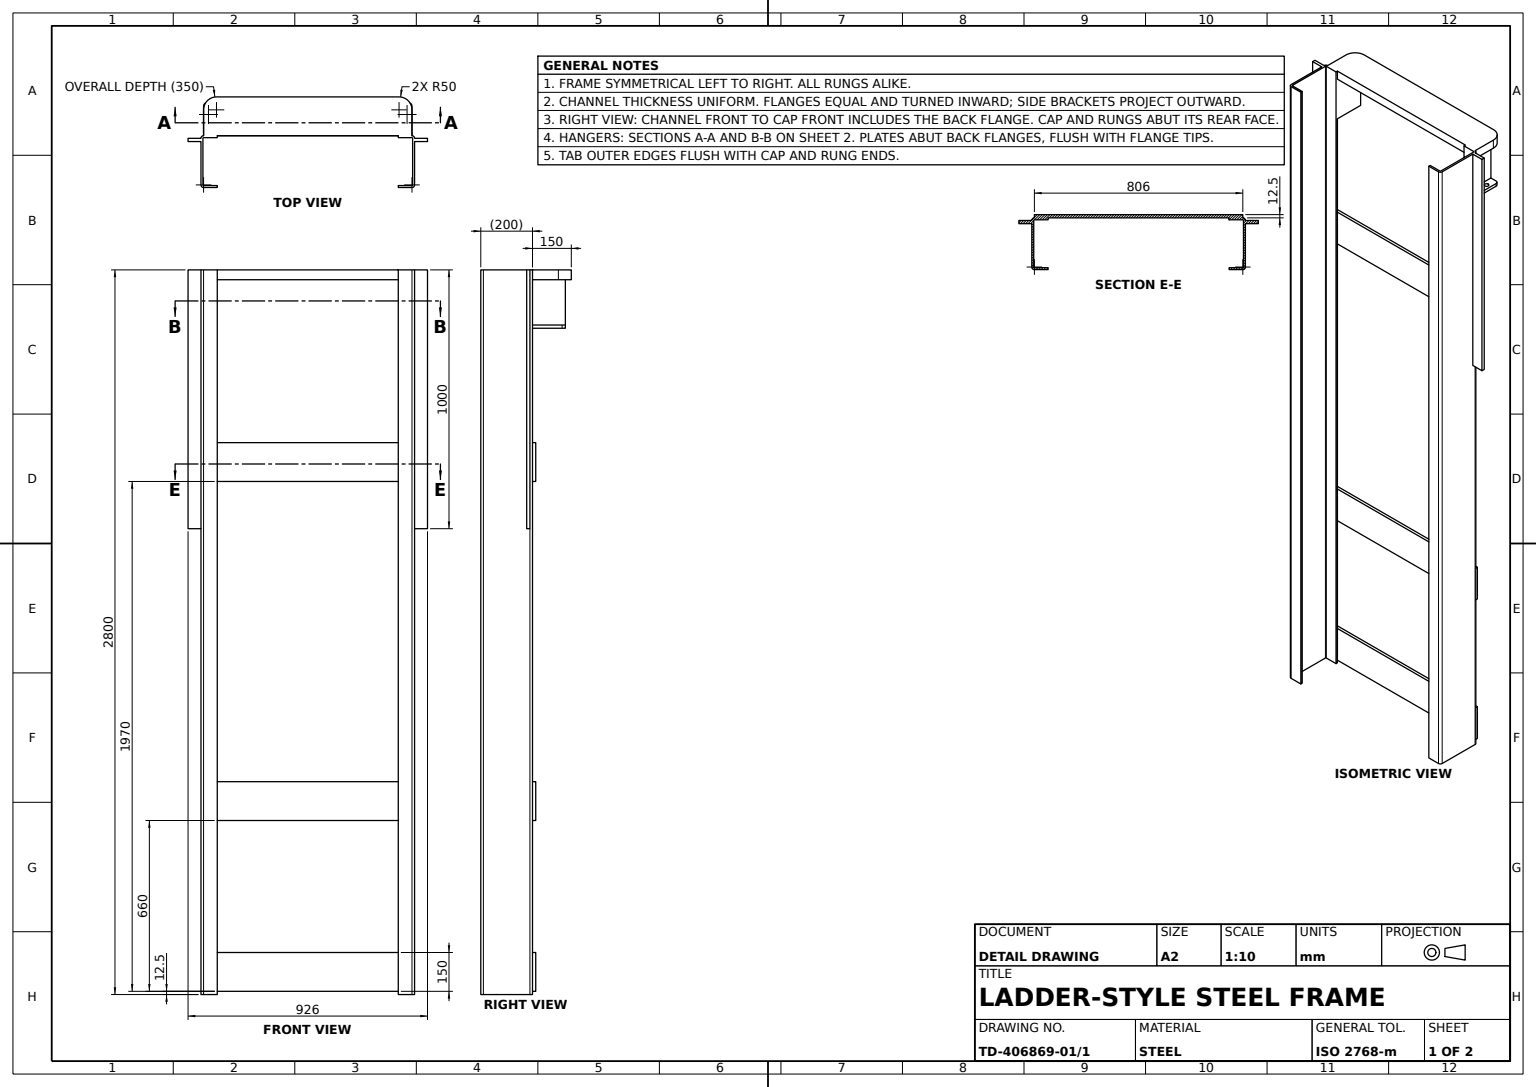
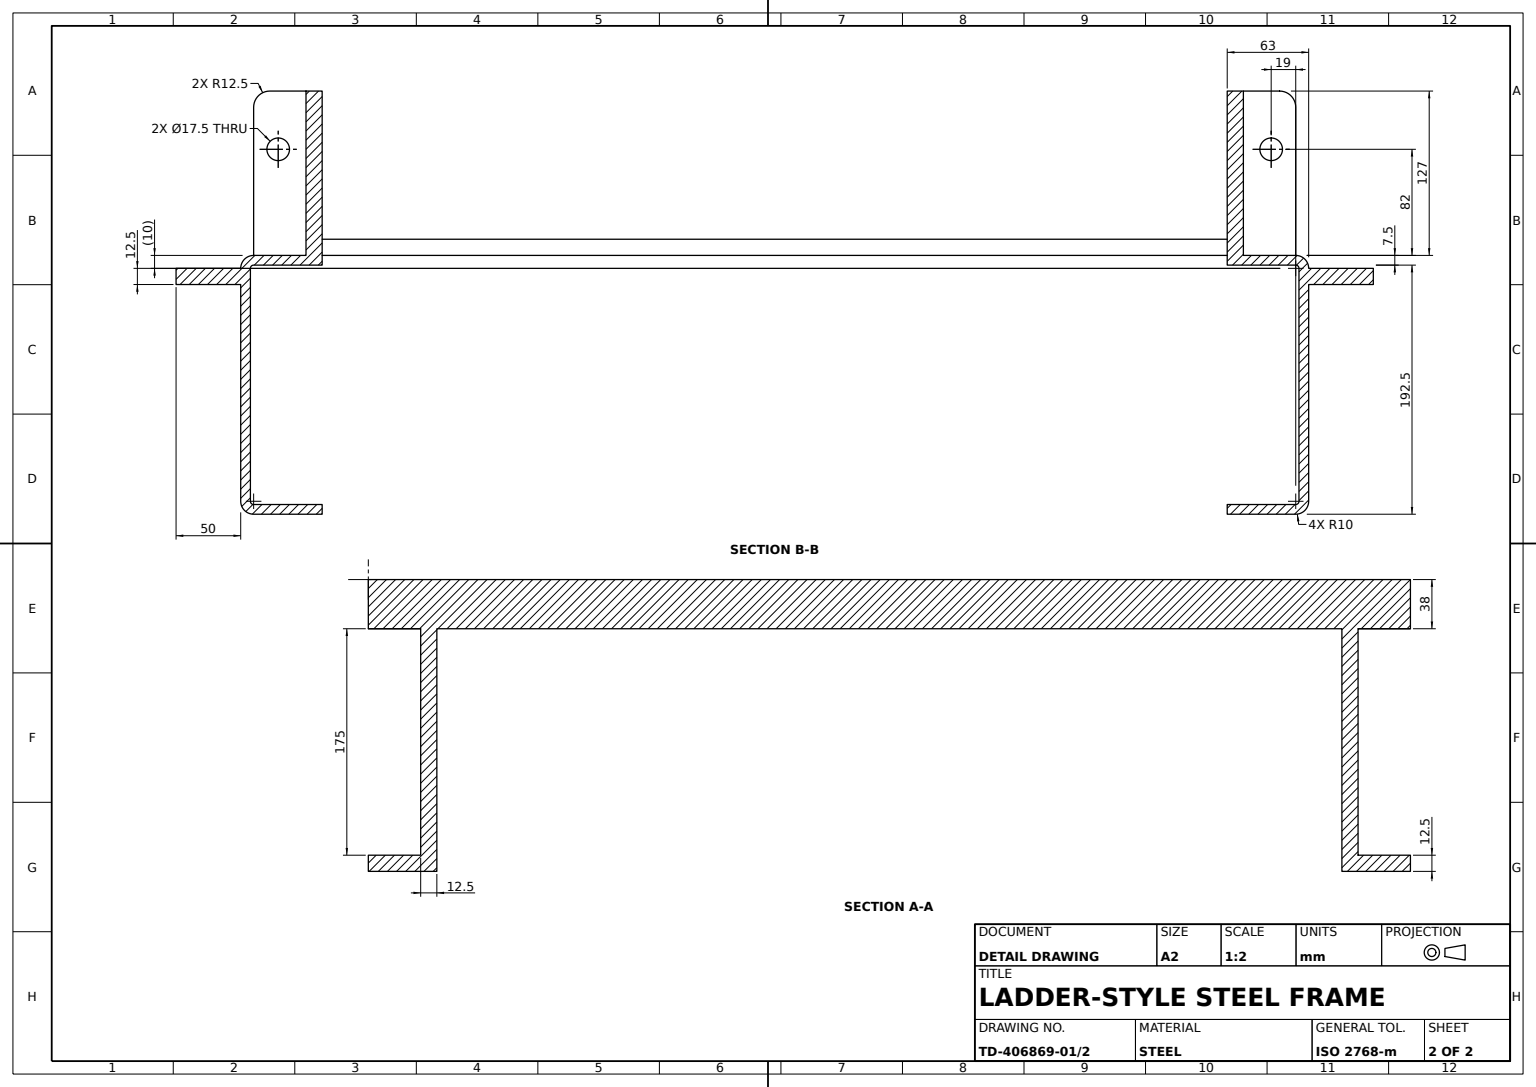
solid
v1 (-403,1400,-200)
v2 (-403,1400,-100)
e1 v1 v2 LINE
v3 (-403,1362,-200)
e2 v3 v1 LINE
v4 (-403,1362,-100)
e3 v3 v4 LINE
e4 v4 v2 LINE
face PLANE(AX(P(-403,1362,-100),D(-1,0,0),D(0,0,1))) [-e1 -e2 e3 e4]
v5 (-350,-1237.5,-100)
v6 (350,-1237.5,-100)
e5 v5 v6 LINE
v7 (-350,-1387.5,-100)
e6 v5 v7 LINE
v8 (350,-1387.5,-100)
e7 v8 v7 LINE
e8 v8 v6 LINE
face PLANE(AX(P(0,0,-100),D(0,0,1),D(1,0,0))) [-e5 e6 -e7 e8]
v9 (384,1174.5,-173.25)
v10 (384,1187,-173.25)
e9 v9 v10 LINE
v11 (384,1187,-190.75)
e10 v10 v11 CIRCLE(AX(P(384,1187,-182),D(0,1,0),D(0,0,-1)),8.75)
v12 (384,1174.5,-190.75)
e11 v12 v11 LINE
e12 v9 v12 CIRCLE(AX(P(384,1174.5,-182),D(0,1,0),D(0,0,-1)),8.75)
face CYL(AX(P(384,1174.5,-182),D(0,1,0),D(0,0,1)),8.75) rev [e9 e10 -e11 -e12]
v13 (350,-727.5,-100)
e13 v13 v6 LINE
v14 (403,-727.5,-100)
e14 v14 v13 LINE
v15 (403,-1237.5,-100)
e15 v14 v15 LINE
e16 v6 v15 LINE
face PLANE(AX(P(350,1400,-100),D(0,0,-1),D(-1,0,0))) [-e13 -e14 e15 -e16]
v16 (-384,1174.5,-173.25)
v17 (-384,1187,-173.25)
e17 v16 v17 LINE
v18 (-384,1174.5,-190.75)
e18 v16 v18 CIRCLE(AX(P(-384,1174.5,-182),D(0,-1,0),D(0,0,-1)),8.75)
v19 (-384,1187,-190.75)
e19 v18 v19 LINE
e20 v17 v19 CIRCLE(AX(P(-384,1187,-182),D(0,-1,0),D(0,0,-1)),8.75)
face CYL(AX(P(-384,1174.5,-182),D(0,1,0),D(0,0,1)),8.75) rev [-e17 e18 e19 -e20]
v20 (390.5,1187,-227)
v21 (362.5,1187,-227)
e21 v20 v21 LINE
v22 (362.5,1187,-100)
e22 v22 v21 LINE
v23 (403,1187,-100)
e23 v22 v23 LINE
v24 (403,1187,-214.5)
e24 v23 v24 LINE
e25 v20 v24 CIRCLE(AX(P(390.5,1187,-214.5),D(0,-1,0),D(0,0,1)),12.5)
e26 v11 v10 CIRCLE(AX(P(384,1187,-182),D(0,1,0),D(0,0,-1)),8.75)
face PLANE(AX(P(0,1187,0),D(0,1,0),D(0,0,1))) [e21 -e22 e23 e24 -e25] [-e26 -e10]
v25 (350,1400,92.5)
v26 (350,-1400,92.5)
e27 v25 v26 LINE
v27 (403,1400,92.5)
e28 v27 v25 LINE
v28 (403,-1400,92.5)
e29 v27 v28 LINE
e30 v28 v26 LINE
face PLANE(AX(P(403,1400,92.5),D(0,0,1),D(1,0,0))) rev [-e27 -e28 e29 e30]
v29 (405.5,1400,90)
e31 v29 v27 CIRCLE(AX(P(403,1400,90),D(0,-1,0),D(1,0,0)),2.5)
v30 (405.5,-1400,90)
e32 v29 v30 LINE
e33 v30 v28 CIRCLE(AX(P(403,-1400,90),D(0,-1,0),D(1,0,0)),2.5)
face CYL(AX(P(403,1400,90),D(0,-1,0),D(0,0,-1)),2.5) rev [-e29 -e31 e32 e33]
v31 (403,1362,-200)
v32 (353,1362,-250)
e34 v31 v32 CIRCLE(AX(P(353,1362,-200),D(0,1,0),D(0,0,-1)),50)
v33 (353,1400,-250)
e35 v32 v33 LINE
v34 (403,1400,-200)
e36 v34 v33 CIRCLE(AX(P(353,1400,-200),D(0,1,0),D(0,0,-1)),50)
e37 v31 v34 LINE
face CYL(AX(P(353,1362,-200),D(0,1,0),D(0,0,1)),50) [e34 e35 -e36 -e37]
v35 (-403,-577.5,-112.5)
v36 (403,-577.5,-112.5)
e38 v35 v36 LINE
v37 (403,-727.5,-112.5)
e39 v36 v37 LINE
v38 (-403,-727.5,-112.5)
e40 v37 v38 LINE
e41 v38 v35 LINE
face PLANE(AX(P(0,660,-112.5),D(0,0,1),D(1,0,0))) rev [e38 e39 e40 e41]
v39 (403,732.5,-112.5)
v40 (403,732.5,-100)
e42 v39 v40 LINE
v41 (403,582.5,-100)
e43 v40 v41 LINE
v42 (403,582.5,-112.5)
e44 v42 v41 LINE
e45 v39 v42 LINE
face PLANE(AX(P(403,582.5,-112.5),D(-1,0,0),D(0,0,1))) rev [e42 e43 -e44 -e45]
v43 (-403,-1237.5,-112.5)
v44 (-403,-1237.5,-100)
e46 v43 v44 LINE
e47 v44 v5 LINE
v45 (403,-1237.5,-112.5)
e48 v45 v15 LINE
e49 v43 v45 LINE
face PLANE(AX(P(403,-1237.5,-112.5),D(0,-1,0),D(0,0,-1))) rev [e46 e47 e5 e16 -e48 -e49]
v46 (-403,-1387.5,-112.5)
v47 (-403,-1387.5,-100)
e50 v46 v47 LINE
e51 v47 v44 LINE
e52 v46 v43 LINE
face PLANE(AX(P(-403,-1387.5,-112.5),D(1,0,0),D(0,0,-1))) rev [e50 e51 -e46 -e52]
v48 (413,-1400,90)
v49 (403,-1400,100)
e53 v48 v49 CIRCLE(AX(P(403,-1400,90),D(0,-1,0),D(0,0,-1)),10)
v50 (413,1400,90)
e54 v50 v48 LINE
v51 (403,1400,100)
e55 v50 v51 CIRCLE(AX(P(403,1400,90),D(0,-1,0),D(0,0,-1)),10)
e56 v51 v49 LINE
face CYL(AX(P(403,1400,90),D(0,-1,0),D(0,0,-1)),10) [-e53 -e54 e55 e56]
v52 (-350,-727.5,-100)
e57 v52 v5 LINE
v53 (-403,-727.5,-100)
e58 v53 v44 LINE
e59 v52 v53 LINE
face PLANE(AX(P(-350,1400,-100),D(0,0,-1),D(1,0,0))) [e57 -e47 -e58 -e59]
e60 v37 v14 LINE
v54 (403,-577.5,-100)
e61 v36 v54 LINE
e62 v54 v14 LINE
face PLANE(AX(P(403,-727.5,-112.5),D(-1,0,0),D(0,0,1))) rev [-e60 -e39 e61 e62]
v55 (-403,1400,92.5)
v56 (-403,-1400,92.5)
e63 v55 v56 LINE
v57 (-405.5,-1400,90)
e64 v57 v56 CIRCLE(AX(P(-403,-1400,90),D(0,1,0),D(-1,0,0)),2.5)
v58 (-405.5,1400,90)
e65 v58 v57 LINE
e66 v58 v55 CIRCLE(AX(P(-403,1400,90),D(0,1,0),D(-1,0,0)),2.5)
face CYL(AX(P(-403,1400,90),D(0,-1,0),D(0,0,-1)),2.5) rev [e63 -e64 -e65 e66]
e67 v38 v53 LINE
v59 (-403,-577.5,-100)
e68 v53 v59 LINE
e69 v35 v59 LINE
face PLANE(AX(P(-403,-727.5,-112.5),D(1,0,0),D(0,0,-1))) rev [-e41 e67 e68 -e69]
e70 v12 v9 CIRCLE(AX(P(384,1174.5,-182),D(0,1,0),D(0,0,-1)),8.75)
face CYL(AX(P(384,1174.5,-182),D(0,1,0),D(0,0,1)),8.75) rev [-e70 e11 e26 -e9]
e71 v18 v16 CIRCLE(AX(P(-384,1174.5,-182),D(0,-1,0),D(0,0,-1)),8.75)
e72 v19 v17 CIRCLE(AX(P(-384,1187,-182),D(0,-1,0),D(0,0,-1)),8.75)
face CYL(AX(P(-384,1174.5,-182),D(0,1,0),D(0,0,1)),8.75) rev [e71 e17 -e72 -e19]
v60 (-390.5,1187,-227)
v61 (-403,1187,-214.5)
e73 v60 v61 CIRCLE(AX(P(-390.5,1187,-214.5),D(0,1,0),D(0,0,1)),12.5)
v62 (-390.5,1174.5,-227)
e74 v62 v60 LINE
v63 (-403,1174.5,-214.5)
e75 v63 v62 CIRCLE(AX(P(-390.5,1174.5,-214.5),D(0,-1,0),D(0,0,1)),12.5)
e76 v61 v63 LINE
face CYL(AX(P(-390.5,1187,-214.5),D(0,1,0),D(0,0,1)),12.5) [-e73 -e74 -e75 -e76]
v64 (413,-1400,-90)
e77 v64 v48 LINE
v65 (413,400,-90)
e78 v65 v64 LINE
v66 (413,400,-77.5)
e79 v65 v66 LINE
v67 (413,1400,-77.5)
e80 v66 v67 LINE
e81 v67 v50 LINE
face PLANE(AX(P(413,1400,-90),D(1,0,0),D(0,0,-1))) [-e77 -e78 e79 e80 e81 e54]
v68 (403,-1400,-92.5)
v69 (405.5,-1400,-90)
e82 v68 v69 CIRCLE(AX(P(403,-1400,-90),D(0,-1,0),D(1,0,0)),2.5)
v70 (405.5,1400,-90)
e83 v70 v69 LINE
v71 (403,1400,-92.5)
e84 v71 v70 CIRCLE(AX(P(403,1400,-90),D(0,-1,0),D(1,0,0)),2.5)
e85 v71 v68 LINE
face CYL(AX(P(403,1400,-90),D(0,-1,0),D(0,0,-1)),2.5) rev [e82 -e83 -e84 e85]
v72 (350,582.5,-100)
v73 (350,732.5,-100)
e86 v72 v73 LINE
v74 (-350,732.5,-100)
e87 v74 v73 LINE
v75 (-350,582.5,-100)
e88 v74 v75 LINE
e89 v72 v75 LINE
face PLANE(AX(P(0,1970,-100),D(0,0,1),D(1,0,0))) [e86 -e87 e88 -e89]
v76 (403,1362,-100)
e90 v76 v31 LINE
v77 (403,1400,-100)
e91 v77 v34 LINE
e92 v77 v76 LINE
face PLANE(AX(P(403,1362,-100),D(1,0,0),D(0,0,-1))) [e90 e37 -e91 e92]
v78 (403,-1387.5,-100)
e93 v78 v8 LINE
v79 (403,-1400,-100)
e94 v78 v79 LINE
v80 (350,-1400,-100)
e95 v80 v79 LINE
e96 v8 v80 LINE
face PLANE(AX(P(350,1400,-100),D(0,0,-1),D(-1,0,0))) [-e93 e94 -e95 -e96]
v81 (403,-1387.5,-112.5)
e97 v81 v46 LINE
e98 v45 v81 LINE
face PLANE(AX(P(0,0,-112.5),D(0,0,1),D(1,0,0))) rev [e97 e52 e49 e98]
v82 (362.5,1362,-100)
e99 v82 v76 LINE
v83 (362.5,1362,-227)
e100 v82 v83 LINE
v84 (350,1362,-227)
e101 v83 v84 LINE
v85 (350,1362,-100)
e102 v84 v85 LINE
v86 (-350,1362,-100)
e103 v86 v85 LINE
v87 (-350,1362,-227)
e104 v87 v86 LINE
v88 (-362.5,1362,-227)
e105 v88 v87 LINE
v89 (-362.5,1362,-100)
e106 v89 v88 LINE
e107 v4 v89 LINE
v90 (-353,1362,-250)
e108 v90 v3 CIRCLE(AX(P(-353,1362,-200),D(0,1,0),D(0,0,-1)),50)
e109 v32 v90 LINE
face PLANE(AX(P(-353,1362,-200),D(0,-1,0),D(0,0,-1))) [-e90 -e99 e100 e101 e102 -e103 -e104 -e105 -e106 -e107 -e3 -e108 -e109 -e34]
v91 (-350,1174.5,-227)
v92 (-350,1174.5,-100)
e110 v91 v92 LINE
v93 (-403,1174.5,-100)
e111 v92 v93 LINE
e112 v93 v63 LINE
e113 v62 v91 LINE
face PLANE(AX(P(0,1174.5,0),D(0,1,0),D(0,0,1))) rev [e110 e111 e112 e75 e113] [-e18 -e71]
v94 (-350,1400,-100)
e114 v94 v86 LINE
v95 (350,1400,-100)
e115 v95 v85 LINE
e116 v94 v95 LINE
face PLANE(AX(P(-403,1362,-100),D(0,0,1),D(1,0,0))) [e114 e103 -e115 -e116]
v96 (-353,1400,-250)
e117 v96 v1 CIRCLE(AX(P(-353,1400,-200),D(0,1,0),D(0,0,-1)),50)
e118 v90 v96 LINE
face CYL(AX(P(-353,1362,-200),D(0,1,0),D(0,0,1)),50) [e108 e2 -e117 -e118]
v97 (-405.5,1400,-90)
e119 v97 v58 LINE
v98 (-405.5,-1400,-90)
e120 v98 v57 LINE
e121 v97 v98 LINE
face PLANE(AX(P(-405.5,1400,-90),D(-1,0,0),D(0,0,-1))) rev [e119 e65 -e120 -e121]
v99 (350,-1400,-92.5)
e122 v99 v80 LINE
e123 v79 v64 CIRCLE(AX(P(403,-1400,-90),D(0,-1,0),D(0,0,-1)),10)
v100 (350,-1400,100)
e124 v49 v100 LINE
e125 v100 v26 LINE
e126 v69 v30 LINE
e127 v99 v68 LINE
face PLANE(AX(P(403,-1400,90),D(0,-1,0),D(-1,0,0))) [e122 e95 e123 e77 e53 e124 e125 -e30 -e33 -e126 -e82 -e127]
v101 (403,1174.5,-214.5)
e128 v24 v101 LINE
v102 (390.5,1174.5,-227)
e129 v101 v102 CIRCLE(AX(P(390.5,1174.5,-214.5),D(0,1,0),D(0,0,1)),12.5)
e130 v102 v20 LINE
face CYL(AX(P(390.5,1187,-214.5),D(0,1,0),D(0,0,1)),12.5) [e25 e128 e129 e130]
v103 (350,-577.5,-100)
e131 v103 v54 LINE
e132 v72 v103 LINE
e133 v41 v72 LINE
e134 v41 v54 LINE
face PLANE(AX(P(350,1400,-100),D(0,0,-1),D(-1,0,0))) [-e131 -e132 -e133 e134]
v104 (463,400,-77.5)
v105 (463,1400,-77.5)
e135 v104 v105 LINE
v106 (463,400,-90)
e136 v104 v106 LINE
v107 (463,1400,-90)
e137 v106 v107 LINE
e138 v105 v107 LINE
face PLANE(AX(P(463,400,-90),D(1,0,0),D(0,0,-1))) [-e135 e136 e137 -e138]
e139 v21 v83 LINE
v108 (350,1174.5,-227)
e140 v102 v108 LINE
e141 v108 v84 LINE
face PLANE(AX(P(350,1187,-227),D(0,0,1),D(-1,0,0))) rev [-e139 -e21 -e130 e140 e141 -e101]
v109 (-403,582.5,-100)
e142 v75 v109 LINE
v110 (-350,-577.5,-100)
e143 v75 v110 LINE
e144 v59 v110 LINE
e145 v109 v59 LINE
face PLANE(AX(P(-350,1400,-100),D(0,0,-1),D(1,0,0))) [-e142 e143 -e144 -e145]
e146 v13 v52 LINE
face PLANE(AX(P(403,-727.5,-112.5),D(0,1,0),D(0,0,1))) rev [e14 e146 e59 -e67 -e40 e60]
v111 (-403,-1400,-100)
e147 v47 v111 LINE
v112 (-413,-1400,-90)
e148 v111 v112 CIRCLE(AX(P(-403,-1400,-90),D(0,1,0),D(0,0,-1)),10)
v113 (-413,400,-90)
e149 v113 v112 LINE
v114 (-413,1400,-90)
e150 v114 v113 LINE
e151 v2 v114 CIRCLE(AX(P(-403,1400,-90),D(0,1,0),D(0,0,-1)),10)
v115 (-403,1187,-100)
e152 v4 v115 LINE
e153 v93 v115 LINE
v116 (-403,732.5,-100)
e154 v93 v116 LINE
e155 v109 v116 LINE
face CYL(AX(P(-403,1400,-90),D(0,-1,0),D(0,0,-1)),10) [e145 -e68 e58 -e51 e147 e148 -e149 -e150 -e151 -e4 e152 -e153 e154 -e155]
v117 (350,1174.5,-100)
e156 v108 v117 LINE
v118 (403,1174.5,-100)
e157 v118 v101 LINE
e158 v117 v118 LINE
face PLANE(AX(P(0,1174.5,0),D(0,1,0),D(0,0,1))) rev [-e156 -e140 -e129 -e157 -e158] [e70 e12]
v119 (-413,1400,-77.5)
v120 (-463,1400,-77.5)
e159 v119 v120 LINE
v121 (-463,400,-77.5)
e160 v121 v120 LINE
v122 (-413,400,-77.5)
e161 v122 v121 LINE
e162 v122 v119 LINE
face PLANE(AX(P(-463,400,-77.5),D(0,0,1),D(-1,0,0))) [e159 -e160 -e161 e162]
e163 v115 v61 LINE
face PLANE(AX(P(-403,1174.5,-100),D(1,0,0),D(0,0,-1))) rev [e163 e76 -e112 e153]
e164 v67 v105 LINE
e165 v66 v104 LINE
face PLANE(AX(P(463,400,-77.5),D(0,0,1),D(1,0,0))) [e135 -e164 -e80 e165]
v123 (-403,-1400,100)
v124 (-350,-1400,100)
e166 v123 v124 LINE
v125 (-350,1400,100)
e167 v125 v124 LINE
v126 (-403,1400,100)
e168 v126 v125 LINE
e169 v126 v123 LINE
face PLANE(AX(P(-403,1400,100),D(0,0,1),D(-1,0,0))) [e166 -e167 -e168 e169]
v127 (-362.5,1187,-100)
e170 v127 v89 LINE
e171 v127 v115 LINE
face PLANE(AX(P(-350,1400,-100),D(0,0,-1),D(1,0,0))) [e107 -e170 e171 -e152]
v128 (-463,400,-90)
e172 v128 v113 LINE
v129 (-463,1400,-90)
e173 v128 v129 LINE
e174 v129 v114 LINE
face PLANE(AX(P(-413,400,-90),D(0,0,-1),D(1,0,0))) [e150 -e172 e173 e174]
e175 v76 v23 LINE
v130 (413,1400,-90)
e176 v77 v130 CIRCLE(AX(P(403,1400,-90),D(0,-1,0),D(0,0,-1)),10)
e177 v130 v65 LINE
e178 v15 v78 LINE
e179 v118 v40 LINE
e180 v118 v23 LINE
face CYL(AX(P(403,1400,-90),D(0,-1,0),D(0,0,-1)),10) [-e175 -e92 e176 e177 e78 -e123 -e94 -e178 -e15 -e62 -e134 -e43 -e179 e180]
v131 (-350,1400,-92.5)
v132 (-350,-1400,-92.5)
e181 v131 v132 LINE
v133 (-403,1400,-92.5)
e182 v131 v133 LINE
v134 (-403,-1400,-92.5)
e183 v133 v134 LINE
e184 v132 v134 LINE
face PLANE(AX(P(-350,1400,-92.5),D(0,0,-1),D(1,0,0))) rev [-e181 e182 e183 -e184]
v135 (-350,-1400,-100)
e185 v7 v135 LINE
e186 v135 v111 LINE
e187 v7 v47 LINE
face PLANE(AX(P(-350,1400,-100),D(0,0,-1),D(1,0,0))) [e185 e186 -e147 -e187]
e188 v73 v40 LINE
v136 (-403,732.5,-112.5)
e189 v136 v39 LINE
e190 v136 v116 LINE
e191 v116 v74 LINE
face PLANE(AX(P(403,732.5,-112.5),D(0,-1,0),D(0,0,-1))) rev [e87 e188 -e42 -e189 e190 e191]
v137 (350,1400,100)
e192 v51 v137 LINE
e193 v137 v100 LINE
face PLANE(AX(P(403,1400,100),D(0,0,1),D(1,0,0))) [e192 e193 -e124 -e56]
e194 v81 v78 LINE
face PLANE(AX(P(403,-1387.5,-112.5),D(0,1,0),D(0,0,1))) rev [-e97 e194 e93 e7 e187 -e50]
e195 v110 v52 LINE
e196 v92 v74 LINE
e197 v91 v87 LINE
e198 v131 v94 LINE
e199 v132 v135 LINE
face PLANE(AX(P(-350,1400,-92.5),D(1,0,0),D(0,0,1))) [-e195 -e143 -e88 -e196 -e110 e197 e104 -e114 -e198 e181 e199 -e185 -e6 -e57]
v138 (-403,582.5,-112.5)
e200 v138 v136 LINE
e201 v42 v138 LINE
face PLANE(AX(P(0,1970,-112.5),D(0,0,1),D(1,0,0))) rev [e200 e189 e45 e201]
v139 (-413,1400,90)
e202 v139 v126 CIRCLE(AX(P(-403,1400,90),D(0,1,0),D(0,0,-1)),10)
v140 (-413,-1400,90)
e203 v139 v140 LINE
e204 v140 v123 CIRCLE(AX(P(-403,-1400,90),D(0,1,0),D(0,0,-1)),10)
face CYL(AX(P(-403,1400,90),D(0,-1,0),D(0,0,-1)),10) [-e202 e203 e204 -e169]
face PLANE(AX(P(403,1174.5,-100),D(-1,0,0),D(0,0,-1))) rev [-e128 -e24 -e180 e157]
e205 v33 v96 LINE
face PLANE(AX(P(-353,1362,-250),D(0,0,-1),D(-1,0,0))) [-e205 -e35 e109 e118]
v141 (-362.5,1187,-227)
e206 v60 v141 LINE
e207 v141 v88 LINE
face PLANE(AX(P(-350,1187,-227),D(0,0,1),D(1,0,0))) rev [e74 e206 e207 e105 -e197 -e113]
e208 v117 v73 LINE
face PLANE(AX(P(350,1400,-100),D(0,0,-1),D(-1,0,0))) [-e208 e158 e179 -e188]
e209 v133 v97 CIRCLE(AX(P(-403,1400,-90),D(0,1,0),D(-1,0,0)),2.5)
e210 v134 v98 CIRCLE(AX(P(-403,-1400,-90),D(0,1,0),D(-1,0,0)),2.5)
face CYL(AX(P(-403,1400,-90),D(0,-1,0),D(0,0,-1)),2.5) rev [-e183 e209 e121 -e210]
e211 v106 v65 LINE
face PLANE(AX(P(0,400,0),D(0,-1,0),D(0,0,-1))) [-e165 -e79 -e211 -e136]
face PLANE(AX(P(403,-1387.5,-112.5),D(-1,0,0),D(0,0,1))) rev [-e194 -e98 e48 e178]
v142 (-350,-1400,92.5)
e212 v56 v142 LINE
e213 v124 v142 LINE
e214 v112 v140 LINE
face PLANE(AX(P(-403,-1400,90),D(0,-1,0),D(1,0,0))) [-e186 -e199 e184 e210 e120 e64 e212 -e213 -e166 -e204 -e214 -e148]
e215 v22 v82 LINE
face PLANE(AX(P(362.5,1187,-100),D(-1,0,0),D(0,0,-1))) rev [-e100 -e215 e22 e139]
v143 (-350,1400,92.5)
e216 v55 v143 LINE
e217 v143 v142 LINE
face PLANE(AX(P(-403,1400,92.5),D(0,0,1),D(-1,0,0))) rev [-e63 e216 e217 -e212]
e218 v107 v130 LINE
face PLANE(AX(P(413,400,-90),D(0,0,-1),D(-1,0,0))) [-e218 -e137 e211 -e177]
v144 (350,1400,-92.5)
e219 v144 v99 LINE
e220 v144 v95 LINE
e221 v13 v103 LINE
face PLANE(AX(P(350,1400,-92.5),D(-1,0,0),D(0,0,1))) [-e219 e220 e115 -e102 -e141 e156 e208 -e86 e132 -e221 e13 -e8 e96 -e122]
e222 v119 v139 LINE
e223 v125 v143 LINE
e224 v144 v71 LINE
e225 v70 v29 LINE
e226 v137 v25 LINE
e227 v120 v129 LINE
face PLANE(AX(P(403,1400,90),D(0,-1,0),D(-1,0,0))) rev [-e159 e222 e202 e168 e223 -e216 -e66 -e119 -e209 -e182 e198 e116 -e220 e224 e84 e225 e31 e28 -e226 -e192 -e55 -e81 e164 e138 e218 -e176 e91 e36 e205 e117 e1 e151 -e174 -e227]
e228 v110 v103 LINE
face PLANE(AX(P(403,-577.5,-112.5),D(0,-1,0),D(0,0,-1))) rev [-e38 e69 e144 e228 e131 -e61]
face PLANE(AX(P(350,1400,-92.5),D(0,0,-1),D(-1,0,0))) rev [e219 e127 -e85 -e224]
e229 v113 v122 LINE
e230 v121 v128 LINE
face PLANE(AX(P(0,400,0),D(0,-1,0),D(0,0,-1))) [e172 e229 e161 e230]
face PLANE(AX(P(-350,1400,-100),D(0,0,-1),D(1,0,0))) [-e154 -e111 e196 -e191]
face PLANE(AX(P(350,1400,-100),D(0,0,-1),D(-1,0,0))) [e99 e175 -e23 e215]
e231 v138 v109 LINE
face PLANE(AX(P(403,582.5,-112.5),D(0,1,0),D(0,0,1))) rev [e142 -e231 -e201 e44 e133 e89]
e232 v127 v141 LINE
face PLANE(AX(P(-362.5,1187,-100),D(1,0,0),D(0,0,-1))) rev [e106 -e207 -e232 e170]
face PLANE(AX(P(405.5,1400,-90),D(1,0,0),D(0,0,-1))) rev [e126 -e32 -e225 e83]
face PLANE(AX(P(0,660,-100),D(0,0,1),D(1,0,0))) [-e146 e221 -e228 e195]
face PLANE(AX(P(-403,582.5,-112.5),D(1,0,0),D(0,0,-1))) rev [-e200 e231 e155 -e190]
face PLANE(AX(P(-413,1400,-90),D(-1,0,0),D(0,0,-1))) [-e229 e149 e214 -e203 -e222 -e162]
face PLANE(AX(P(-350,1400,100),D(1,0,0),D(0,0,1))) [e167 e213 -e217 -e223]
face PLANE(AX(P(350,1400,100),D(-1,0,0),D(0,0,1))) [-e193 e226 e27 -e125]
face PLANE(AX(P(0,1187,0),D(0,1,0),D(0,0,1))) [e20 e72] [-e206 e73 -e163 -e171 e232]
face PLANE(AX(P(-463,400,-90),D(-1,0,0),D(0,0,-1))) [e160 e227 -e173 -e230]
